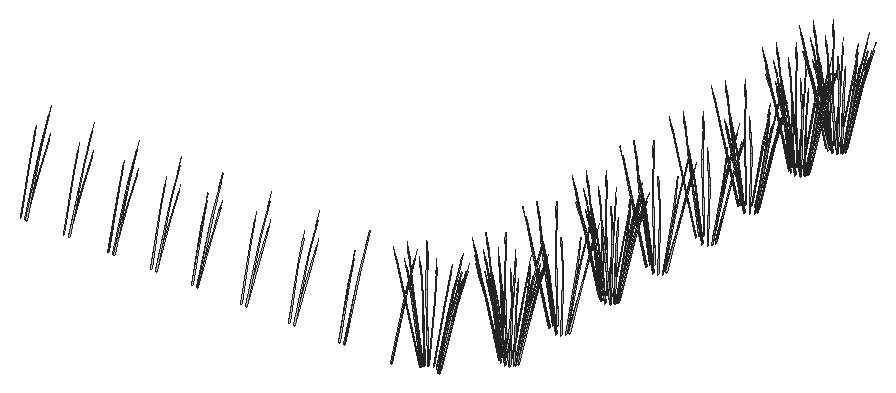
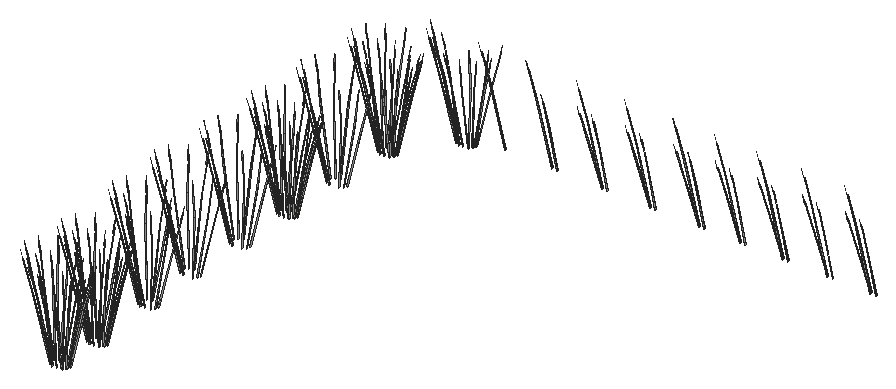
# SketchUp Ruby script. Lengths in inches.
U = 1.inch
M = Sketchup.active_model
def pt(a) = Geom::Point3d.new(a.map { |v| v * U })
def face(e, loops, mat)
  f = e.add_face(loops[0].map { |a| pt(a) })
  loops[1..].each { |l| e.add_face(l.map { |a| pt(a) }).erase! }
  f.material = f.back_material = mat if mat
  f
end
# faces: each face lists its corners as indices into pts; further lists are holes
def faces(e, pts, list, mat = nil) = list.each { |f| face(e, (f[0].is_a?(Array) ? f : [f]).map { |l| l.map { |i| pts[i] } }, mat) }
# xy, xz, yz: faces in a plane at the given z, y or x. An outline is a flat list of corners, or four numbers for a rectangle; further outlines are holes
def ring(l) = l.size == 4 ? [[l[0], l[1]], [l[2], l[1]], [l[2], l[3]], [l[0], l[3]]] : l.each_slice(2).to_a
def flat(e, list, mat, &to3) = list.each { |f| face(e, (f[0].is_a?(Array) ? f : [f]).map { |l| ring(l).map { |u, v| to3.(u, v) } }, mat) }
def xy(e, z, list, mat = nil) = flat(e, list, mat) { |x, y| [x, y, z] }
def xz(e, y, list, mat = nil) = flat(e, list, mat) { |x, z| [x, y, z] }
def yz(e, x, list, mat = nil) = flat(e, list, mat) { |y, z| [x, y, z] }
def lines(e, pts, list) = list.each { |a, b| e.add_line(pt(pts[a]), pt(pts[b])) }
# prism: a flat outline (further loops are holes) pulled along v
def prism(e, loops, v, mat = nil)
  f = face(e, loops, mat); d = Geom::Vector3d.new(v.map { |x| x * U })
  f.pushpull(f.normal.samedirection?(d) ? d.length : -d.length)
end
def box(e, o, s, mat = nil) = prism(e, [[o, [o[0] + s[0], o[1], o[2]], [o[0] + s[0], o[1] + s[1], o[2]], [o[0], o[1] + s[1], o[2]]]], [0, 0, s[2]], mat)
def at(x, y, z, deg = 0) = Geom::Transformation.translation(pt([x, y, z])) * Geom::Transformation.rotation(ORIGIN, Z_AXIS, deg.degrees)
def axes(o, x, y, z) = Geom::Transformation.new([*x, 0, *y, 0, *z, 0, *pt(o).to_a, 1])
def part(name) = M.definitions.add(name)
# library, detail: a bought-in or finely detailed component or shape, given as its bounding box
def library(name, o, s) = part(name).tap { |d| box(d.entities, o, s) }
def detail(e, o, s) = box(e.add_group.entities, o, s)
def put(e, d, t, mat = nil) = e.add_instance(d, t).tap { |i| i.material = mat if mat }
def group(e, t, mat = nil) = e.add_group.tap { |g| g.transformation = t; g.material = mat if mat }.entities
root = M.entities
M.materials.add("LightPink_Translucent").color = [144, 107, 117]
M.materials["LightPink_Translucent"].alpha = 0.75
c1 = part("blade")
p = [[2.15,0.21,22],[0,0.17,0],[0.09,0.45,0],[2.18,0.31,22],[2.29,0.31,22],[0.38,0.45,0],
  [2.48,0.24,33],[2.49,0.24,33],[2.48,0.22,33]]
faces(c1.entities,p,[[0,1,2,3],[4,5,2,3],[6,3,4,7],[8,0,3,6]])
c2 = part("seeds")
p = [[0.3,-0.1,1.38],[-0.01,-0.03,1.59],[-0.01,-0.03,0.03],[0.14,-0.07,-0.07],[0.29,-0.03,3],[0.15,0.01,3.11]]
faces(c2.entities,p,[[0,1,2,3],[1,0,4,5]],"LightPink_Translucent")
c3 = part("blade with seeds")
put(c3.entities,c1,at(0,0,0))
put(c3.entities,c2,axes([2.4,0.25,30.99],[1.5799,-0.05474,1.17369],[-0.12525,1.92788,0.29478],[-0.07173,-0.02425,1.56792]))
put(root,c3,axes([346.88,56.26,259.73],[-0.34533,0.38816,0.0643],[-0.49176,-0.22599,0.50621],[0.15898,0.12445,0.77189]))
put(root,c3,axes([328.97,56.26,259.73],[-0.34533,0.38816,0.0643],[-0.49176,-0.22599,0.50621],[0.15898,0.12445,0.77189]))
put(root,c3,axes([310.87,56.26,259.73],[-0.34533,0.38816,0.0643],[-0.49176,-0.22599,0.50621],[0.15898,0.12445,0.77189]))
put(root,c3,axes([295.42,56.26,259.73],[-0.34533,0.38816,0.0643],[-0.49176,-0.22599,0.50621],[0.15898,0.12445,0.77189]))
put(root,c3,axes([279.69,56.26,259.73],[-0.34533,0.38816,0.0643],[-0.49176,-0.22599,0.50621],[0.15898,0.12445,0.77189]))
put(root,c3,axes([262.96,56.26,259.73],[-0.34533,0.38816,0.0643],[-0.49176,-0.22599,0.50621],[0.15898,0.12445,0.77189]))
put(root,c3,axes([246.9,56.26,259.73],[-0.34533,0.38816,0.0643],[-0.49176,-0.22599,0.50621],[0.15898,0.12445,0.77189]))
put(root,c3,axes([397.37,60.31,260.05],[-0.63144,-0.17046,0.35414],[0.18417,-0.49731,-0.4572],[0.25423,-0.0456,0.87481]))
put(root,c3,axes([383.44,56.15,259.73],[-0.75571,0.14023,0.48003],[-0.13115,-0.55007,0.3958],[0.17773,0.16212,0.9933]))
put(root,c3,axes([365.81,56.15,259.73],[-0.75571,0.14023,0.48003],[-0.13115,-0.55007,0.3958],[0.17773,0.16212,0.9933]))
put(root,c3,axes([347.03,56.15,259.73],[-0.75571,0.14023,0.48003],[-0.13115,-0.55007,0.3958],[0.17773,0.16212,0.9933]))
put(root,c3,axes([329.12,56.15,259.73],[-0.75571,0.14023,0.48003],[-0.13115,-0.55007,0.3958],[0.17773,0.16212,0.9933]))
put(root,c3,axes([311.01,56.15,259.73],[-0.75571,0.14023,0.48003],[-0.13115,-0.55007,0.3958],[0.17773,0.16212,0.9933]))
put(root,c3,axes([295.5625,56.15,259.73],[-0.75571,0.14023,0.48003],[-0.13115,-0.55007,0.3958],[0.17773,0.16212,0.9933]))
put(root,c3,axes([279.84,56.15,259.73],[-0.75571,0.14023,0.48003],[-0.13115,-0.55007,0.3958],[0.17773,0.16212,0.9933]))
put(root,c3,axes([263.11,56.15,259.73],[-0.75571,0.14023,0.48003],[-0.13115,-0.55007,0.3958],[0.17773,0.16212,0.9933]))
put(root,c3,axes([247.04,56.15,259.73],[-0.75571,0.14023,0.48003],[-0.13115,-0.55007,0.3958],[0.17773,0.16212,0.9933]))
put(root,c3,axes([390.76,59.4,259.73],[0.21466,-0.55714,0.48003],[0.70573,0.19051,0.3958],[-0.27753,0.03348,0.9933]))
put(root,c3,axes([363.75,56.32,259.73],[-0.55987,0.20767,0.0643],[-0.27403,-0.37869,0.50621],[0.05407,0.16693,0.77189]))
put(root,c3,axes([344.96,56.32,259.73],[-0.55987,0.20767,0.0643],[-0.27403,-0.37869,0.50621],[0.05407,0.16693,0.77189]))
put(root,c3,axes([327.06,56.32,259.73],[-0.55987,0.20767,0.0643],[-0.27403,-0.37869,0.50621],[0.05407,0.16693,0.77189]))
put(root,c3,axes([308.95,56.32,259.73],[-0.55987,0.20767,0.0643],[-0.27403,-0.37869,0.50621],[0.05407,0.16693,0.77189]))
put(root,c3,axes([293.5,56.32,259.73],[-0.55987,0.20767,0.0643],[-0.27403,-0.37869,0.50621],[0.05407,0.16693,0.77189]))
put(root,c3,axes([277.77,56.32,259.73],[-0.55987,0.20767,0.0643],[-0.27403,-0.37869,0.50621],[0.05407,0.16693,0.77189]))
put(root,c3,axes([261.04,56.32,259.73],[-0.55987,0.20767,0.0643],[-0.27403,-0.37869,0.50621],[0.05407,0.16693,0.77189]))
put(root,c3,axes([244.98,56.32,259.73],[-0.55987,0.20767,0.0643],[-0.27403,-0.37869,0.50621],[0.05407,0.16693,0.77189]))
put(root,c3,axes([397.89,60.3125,259.73],[-0.21466,0.55714,0.48003],[-0.70573,-0.19051,0.3958],[0.27753,-0.03348,0.9933]))
put(root,c3,axes([391.28,59.4,260.05],[0.63144,0.17046,0.35414],[-0.18417,0.49731,-0.4572],[-0.25423,0.0456,0.87481]))
put(root,c3,axes([396.66,61.38,260.05],[-0.43232,-0.38257,0.35414],[0.49364,-0.36215,-0.4572],[0.25081,0.0551,0.87481]))
put(root,c3,axes([390.93,60.78,259.73],[-0.18844,-0.56237,0.48003],[0.73919,-0.0976,0.3958],[-0.21785,0.13226,0.9933]))
put(root,c3,axes([391.39,60.6,260.05],[0.66138,-0.08733,0.35414],[0.17464,0.49921,-0.4572],[-0.18953,0.13408,0.87481]))
put(root,c3,axes([397.11,61.58,259.73],[-0.56024,0.40262,0.48003],[-0.48318,-0.42758,0.3958],[0.26285,0.07427,0.9933]))
put(root,c3,axes([395.32,62.04,260.05],[-0.11735,-0.49217,0.35414],[0.67083,-0.12996,-0.4572],[0.18018,0.14104,0.87481]))
put(root,c3,axes([392.28,61.59,260.05],[0.5141,-0.32171,0.35414],[0.48666,0.36734,-0.4572],[-0.07405,0.18664,0.87481]))
put(root,c3,axes([392.01,61.92,259.73],[-0.54105,-0.41691,0.48003],[0.57458,-0.35956,0.3958],[-0.0998,0.1956,0.9933]))
put(root,c3,axes([393.72,62.12,260.05],[0.22906,-0.4699,0.35414],[0.66828,0.13705,-0.4572],[0.06128,0.18919,0.87481]))
put(root,c3,axes([395.58,62.38,259.73],[-0.75571,0.14023,0.48003],[-0.13115,-0.55007,0.3958],[0.17773,0.16212,0.9933]))
put(root,c3,axes([409.56,75.64,259.73],[0.74868,0.15974,0.48003],[-0.25601,0.52518,0.3958],[-0.04499,-0.20653,0.9933]))
put(root,c3,axes([409.55,76.02,260.05],[-0.22906,0.4699,0.35414],[-0.66828,-0.13705,-0.4572],[-0.06128,-0.18919,0.87481]))
put(root,c3,axes([411.26,76.22,259.73],[0.54105,0.41691,0.48003],[-0.57458,0.35956,0.3958],[0.0998,-0.1956,0.9933]))
put(root,c3,axes([410.99,76.55,260.05],[-0.5141,0.32171,0.35414],[-0.48666,-0.36734,-0.4572],[0.07405,-0.18664,0.87481]))
put(root,c3,axes([407.94,76.1,260.05],[0.11735,0.49217,0.35414],[-0.67083,0.12996,-0.4572],[-0.18018,-0.14104,0.87481]))
put(root,c3,axes([411.88,77.55,260.05],[-0.66138,0.08733,0.35414],[-0.17464,-0.49921,-0.4572],[0.18953,-0.13408,0.87481]))
put(root,c3,axes([412.34,77.36,259.73],[0.18844,0.56237,0.48003],[-0.73919,0.0976,0.3958],[0.21785,-0.13226,0.9933]))
put(root,c3,axes([406.61,76.77,260.05],[0.43232,0.38257,0.35414],[-0.49364,0.36215,-0.4572],[-0.25081,-0.0551,0.87481]))
put(root,c3,axes([411.99,78.74,260.05],[-0.63144,-0.17046,0.35414],[0.18417,-0.49731,-0.4572],[0.25423,-0.0456,0.87481]))
put(root,c3,axes([405.38,77.83,259.73],[0.21466,-0.55714,0.48003],[0.70573,0.19051,0.3958],[-0.27753,0.03348,0.9933]))
put(root,c3,axes([412.51,78.75,259.73],[-0.21466,0.55714,0.48003],[-0.70573,-0.19051,0.3958],[0.27753,-0.03348,0.9933]))
put(root,c3,axes([405.9,77.84,260.05],[0.63144,0.17046,0.35414],[-0.18417,0.49731,-0.4572],[-0.25423,0.0456,0.87481]))
put(root,c3,axes([411.28,79.8125,260.05],[-0.43232,-0.38257,0.35414],[0.49364,-0.36215,-0.4572],[0.25081,0.0551,0.87481]))
put(root,c3,axes([405.55,79.22,259.73],[-0.18844,-0.56237,0.48003],[0.73919,-0.0976,0.3958],[-0.21785,0.13226,0.9933]))
put(root,c3,axes([406,79.03,260.05],[0.66138,-0.08733,0.35414],[0.17464,0.49921,-0.4572],[-0.18953,0.13408,0.87481]))
put(root,c3,axes([411.72,80.01,259.73],[-0.56024,0.40262,0.48003],[-0.48318,-0.42758,0.3958],[0.26285,0.07427,0.9933]))
put(root,c3,axes([409.94,80.48,260.05],[-0.11735,-0.49217,0.35414],[0.67083,-0.12996,-0.4572],[0.18018,0.14104,0.87481]))
put(root,c3,axes([406.89,80.03,260.05],[0.5141,-0.32171,0.35414],[0.48666,0.36734,-0.4572],[-0.07405,0.18664,0.87481]))
put(root,c3,axes([406.63,80.36,259.73],[-0.54105,-0.41691,0.48003],[0.57458,-0.35956,0.3958],[-0.0998,0.1956,0.9933]))
put(root,c3,axes([408.34,80.56,260.05],[0.22906,-0.4699,0.35414],[0.66828,0.13705,-0.4572],[0.06128,0.18919,0.87481]))
put(root,c3,axes([410.19,80.81,259.73],[-0.75571,0.14023,0.48003],[-0.13115,-0.55007,0.3958],[0.17773,0.16212,0.9933]))
put(root,c3,axes([409.68,99.16,259.73],[0.74868,0.15974,0.48003],[-0.25601,0.52518,0.3958],[-0.04499,-0.20653,0.9933]))
put(root,c3,axes([411.38,99.75,259.73],[0.54105,0.41691,0.48003],[-0.57458,0.35956,0.3958],[0.0998,-0.1956,0.9933]))
put(root,c3,axes([412.46,100.89,259.73],[0.18844,0.56237,0.48003],[-0.73919,0.0976,0.3958],[0.21785,-0.13226,0.9933]))
put(root,c3,axes([405.5,101.36,259.73],[0.21466,-0.55714,0.48003],[0.70573,0.19051,0.3958],[-0.27753,0.03348,0.9933]))
put(root,c3,axes([412.63,102.27,259.73],[-0.21466,0.55714,0.48003],[-0.70573,-0.19051,0.3958],[0.27753,-0.03348,0.9933]))
put(root,c3,axes([405.67,102.74,259.73],[-0.18844,-0.56237,0.48003],[0.73919,-0.0976,0.3958],[-0.21785,0.13226,0.9933]))
put(root,c3,axes([411.85,103.54,259.73],[-0.56024,0.40262,0.48003],[-0.48318,-0.42758,0.3958],[0.26285,0.07427,0.9933]))
put(root,c3,axes([406.75,103.88,259.73],[-0.54105,-0.41691,0.48003],[0.57458,-0.35956,0.3958],[-0.0998,0.1956,0.9933]))
put(root,c3,axes([410.32,104.34,259.73],[-0.75571,0.14023,0.48003],[-0.13115,-0.55007,0.3958],[0.17773,0.16212,0.9933]))
put(root,c3,axes([409.46,122.55,259.73],[0.74868,0.15974,0.48003],[-0.25601,0.52518,0.3958],[-0.04499,-0.20653,0.9933]))
put(root,c3,axes([409.46,122.94,260.05],[-0.22906,0.4699,0.35414],[-0.66828,-0.13705,-0.4572],[-0.06128,-0.18919,0.87481]))
put(root,c3,axes([411.16,123.13,259.73],[0.54105,0.41691,0.48003],[-0.57458,0.35956,0.3958],[0.0998,-0.1956,0.9933]))
put(root,c3,axes([410.9,123.46,260.05],[-0.5141,0.32171,0.35414],[-0.48666,-0.36734,-0.4572],[0.07405,-0.18664,0.87481]))
put(root,c3,axes([407.85,123.01,260.05],[0.11735,0.49217,0.35414],[-0.67083,0.12996,-0.4572],[-0.18018,-0.14104,0.87481]))
put(root,c3,axes([411.79,124.46,260.05],[-0.66138,0.08733,0.35414],[-0.17464,-0.49921,-0.4572],[0.18953,-0.13408,0.87481]))
put(root,c3,axes([412.24,124.27,259.73],[0.18844,0.56237,0.48003],[-0.73919,0.0976,0.3958],[0.21785,-0.13226,0.9933]))
put(root,c3,axes([406.51,123.68,260.05],[0.43232,0.38257,0.35414],[-0.49364,0.36215,-0.4572],[-0.25081,-0.0551,0.87481]))
put(root,c3,axes([411.9,125.65,260.05],[-0.63144,-0.17046,0.35414],[0.18417,-0.49731,-0.4572],[0.25423,-0.0456,0.87481]))
put(root,c3,axes([405.28,124.74,259.73],[0.21466,-0.55714,0.48003],[0.70573,0.19051,0.3958],[-0.27753,0.03348,0.9933]))
put(root,c3,axes([412.41,125.66,259.73],[-0.21466,0.55714,0.48003],[-0.70573,-0.19051,0.3958],[0.27753,-0.03348,0.9933]))
put(root,c3,axes([405.8,124.75,260.05],[0.63144,0.17046,0.35414],[-0.18417,0.49731,-0.4572],[-0.25423,0.0456,0.87481]))
put(root,c3,axes([411.18,126.73,260.05],[-0.43232,-0.38257,0.35414],[0.49364,-0.36215,-0.4572],[0.25081,0.0551,0.87481]))
put(root,c3,axes([405.45,126.13,259.73],[-0.18844,-0.56237,0.48003],[0.73919,-0.0976,0.3958],[-0.21785,0.13226,0.9933]))
put(root,c3,axes([405.91,125.94,260.05],[0.66138,-0.08733,0.35414],[0.17464,0.49921,-0.4572],[-0.18953,0.13408,0.87481]))
put(root,c3,axes([411.63,126.92,259.73],[-0.56024,0.40262,0.48003],[-0.48318,-0.42758,0.3958],[0.26285,0.07427,0.9933]))
put(root,c3,axes([409.85,127.39,260.05],[-0.11735,-0.49217,0.35414],[0.67083,-0.12996,-0.4572],[0.18018,0.14104,0.87481]))
put(root,c3,axes([406.8,126.9375,260.05],[0.5141,-0.32171,0.35414],[0.48666,0.36734,-0.4572],[-0.07405,0.18664,0.87481]))
put(root,c3,axes([406.53,127.27,259.73],[-0.54105,-0.41691,0.48003],[0.57458,-0.35956,0.3958],[-0.0998,0.1956,0.9933]))
put(root,c3,axes([408.24,127.47,260.05],[0.22906,-0.4699,0.35414],[0.66828,0.13705,-0.4572],[0.06128,0.18919,0.87481]))
put(root,c3,axes([410.1,127.73,259.73],[-0.75571,0.14023,0.48003],[-0.13115,-0.55007,0.3958],[0.17773,0.16212,0.9933]))
put(root,c3,axes([409.1875,144.96,259.73],[0.74868,0.15974,0.48003],[-0.25601,0.52518,0.3958],[-0.04499,-0.20653,0.9933]))
put(root,c3,axes([410.89,145.54,259.73],[0.54105,0.41691,0.48003],[-0.57458,0.35956,0.3958],[0.0998,-0.1956,0.9933]))
put(root,c3,axes([411.97,146.68,259.73],[0.18844,0.56237,0.48003],[-0.73919,0.0976,0.3958],[0.21785,-0.13226,0.9933]))
put(root,c3,axes([405.01,147.15,259.73],[0.21466,-0.55714,0.48003],[0.70573,0.19051,0.3958],[-0.27753,0.03348,0.9933]))
put(root,c3,axes([412.14,148.07,259.73],[-0.21466,0.55714,0.48003],[-0.70573,-0.19051,0.3958],[0.27753,-0.03348,0.9933]))
put(root,c3,axes([405.18,148.54,259.73],[-0.18844,-0.56237,0.48003],[0.73919,-0.0976,0.3958],[-0.21785,0.13226,0.9933]))
put(root,c3,axes([411.35,149.33,259.73],[-0.56024,0.40262,0.48003],[-0.48318,-0.42758,0.3958],[0.26285,0.07427,0.9933]))
put(root,c3,axes([406.26,149.68,259.73],[-0.54105,-0.41691,0.48003],[0.57458,-0.35956,0.3958],[-0.0998,0.1956,0.9933]))
put(root,c3,axes([409.82,150.14,259.73],[-0.75571,0.14023,0.48003],[-0.13115,-0.55007,0.3958],[0.17773,0.16212,0.9933]))
put(root,c3,axes([409.55,167.55,259.73],[0.74868,0.15974,0.48003],[-0.25601,0.52518,0.3958],[-0.04499,-0.20653,0.9933]))
put(root,c3,axes([411.25,168.14,259.73],[0.54105,0.41691,0.48003],[-0.57458,0.35956,0.3958],[0.0998,-0.1956,0.9933]))
put(root,c3,axes([412.33,169.28,259.73],[0.18844,0.56237,0.48003],[-0.73919,0.0976,0.3958],[0.21785,-0.13226,0.9933]))
put(root,c3,axes([405.37,169.75,259.73],[0.21466,-0.55714,0.48003],[0.70573,0.19051,0.3958],[-0.27753,0.03348,0.9933]))
put(root,c3,axes([412.5,170.66,259.73],[-0.21466,0.55714,0.48003],[-0.70573,-0.19051,0.3958],[0.27753,-0.03348,0.9933]))
put(root,c3,axes([405.54,171.14,259.73],[-0.18844,-0.56237,0.48003],[0.73919,-0.0976,0.3958],[-0.21785,0.13226,0.9933]))
put(root,c3,axes([411.71,171.93,259.73],[-0.56024,0.40262,0.48003],[-0.48318,-0.42758,0.3958],[0.26285,0.07427,0.9933]))
put(root,c3,axes([406.62,172.27,259.73],[-0.54105,-0.41691,0.48003],[0.57458,-0.35956,0.3958],[-0.0998,0.1956,0.9933]))
put(root,c3,axes([410.18,172.73,259.73],[-0.75571,0.14023,0.48003],[-0.13115,-0.55007,0.3958],[0.17773,0.16212,0.9933]))
put(root,c3,axes([407.53,189.68,259.73],[0.74868,0.15974,0.48003],[-0.25601,0.52518,0.3958],[-0.04499,-0.20653,0.9933]))
put(root,c3,axes([407.52,190.07,260.05],[-0.22906,0.4699,0.35414],[-0.66828,-0.13705,-0.4572],[-0.06128,-0.18919,0.87481]))
put(root,c3,axes([409.23,190.27,259.73],[0.54105,0.41691,0.48003],[-0.57458,0.35956,0.3958],[0.0998,-0.1956,0.9933]))
put(root,c3,axes([410.31,191.41,259.73],[0.18844,0.56237,0.48003],[-0.73919,0.0976,0.3958],[0.21785,-0.13226,0.9933]))
put(root,c3,axes([409.96,192.79,260.05],[-0.63144,-0.17046,0.35414],[0.18417,-0.49731,-0.4572],[0.25423,-0.0456,0.87481]))
put(root,c3,axes([403.35,191.88,259.73],[0.21466,-0.55714,0.48003],[0.70573,0.19051,0.3958],[-0.27753,0.03348,0.9933]))
put(root,c3,axes([410.48,192.79,259.73],[-0.21466,0.55714,0.48003],[-0.70573,-0.19051,0.3958],[0.27753,-0.03348,0.9933]))
put(root,c3,axes([409.25,193.86,260.05],[-0.43232,-0.38257,0.35414],[0.49364,-0.36215,-0.4572],[0.25081,0.0551,0.87481]))
put(root,c3,axes([403.52,193.27,259.73],[-0.18844,-0.56237,0.48003],[0.73919,-0.0976,0.3958],[-0.21785,0.13226,0.9933]))
put(root,c3,axes([409.69,194.06,259.73],[-0.56024,0.40262,0.48003],[-0.48318,-0.42758,0.3958],[0.26285,0.07427,0.9933]))
put(root,c3,axes([404.6,194.4,259.73],[-0.54105,-0.41691,0.48003],[0.57458,-0.35956,0.3958],[-0.0998,0.1956,0.9933]))
put(root,c3,axes([406.31,194.6,260.05],[0.22906,-0.4699,0.35414],[0.66828,0.13705,-0.4572],[0.06128,0.18919,0.87481]))
put(root,c3,axes([408.16,194.86,259.73],[-0.75571,0.14023,0.48003],[-0.13115,-0.55007,0.3958],[0.17773,0.16212,0.9933]))
put(root,c3,axes([405.125,216.4375,259.73],[0.74868,0.15974,0.48003],[-0.25601,0.52518,0.3958],[-0.04499,-0.20653,0.9933]))
put(root,c3,axes([405.12,216.82,260.05],[-0.22906,0.4699,0.35414],[-0.66828,-0.13705,-0.4572],[-0.06128,-0.18919,0.87481]))
put(root,c3,axes([406.83,217.02,259.73],[0.54105,0.41691,0.48003],[-0.57458,0.35956,0.3958],[0.0998,-0.1956,0.9933]))
put(root,c3,axes([406.56,217.35,260.05],[-0.5141,0.32171,0.35414],[-0.48666,-0.36734,-0.4572],[0.07405,-0.18664,0.87481]))
put(root,c3,axes([403.51,216.9,260.05],[0.11735,0.49217,0.35414],[-0.67083,0.12996,-0.4572],[-0.18018,-0.14104,0.87481]))
put(root,c3,axes([407.45,218.35,260.05],[-0.66138,0.08733,0.35414],[-0.17464,-0.49921,-0.4572],[0.18953,-0.13408,0.87481]))
put(root,c3,axes([407.91,218.16,259.73],[0.18844,0.56237,0.48003],[-0.73919,0.0976,0.3958],[0.21785,-0.13226,0.9933]))
put(root,c3,axes([402.18,217.57,260.05],[0.43232,0.38257,0.35414],[-0.49364,0.36215,-0.4572],[-0.25081,-0.0551,0.87481]))
put(root,c3,axes([407.56,219.54,260.05],[-0.63144,-0.17046,0.35414],[0.18417,-0.49731,-0.4572],[0.25423,-0.0456,0.87481]))
put(root,c3,axes([400.95,218.63,259.73],[0.21466,-0.55714,0.48003],[0.70573,0.19051,0.3958],[-0.27753,0.03348,0.9933]))
put(root,c3,axes([408.08,219.55,259.73],[-0.21466,0.55714,0.48003],[-0.70573,-0.19051,0.3958],[0.27753,-0.03348,0.9933]))
put(root,c3,axes([401.46,218.64,260.05],[0.63144,0.17046,0.35414],[-0.18417,0.49731,-0.4572],[-0.25423,0.0456,0.87481]))
put(root,c3,axes([406.85,220.61,260.05],[-0.43232,-0.38257,0.35414],[0.49364,-0.36215,-0.4572],[0.25081,0.0551,0.87481]))
put(root,c3,axes([401.12,220.02,259.73],[-0.18844,-0.56237,0.48003],[0.73919,-0.0976,0.3958],[-0.21785,0.13226,0.9933]))
put(root,c3,axes([401.57,219.83,260.05],[0.66138,-0.08733,0.35414],[0.17464,0.49921,-0.4572],[-0.18953,0.13408,0.87481]))
put(root,c3,axes([407.29,220.8125,259.73],[-0.56024,0.40262,0.48003],[-0.48318,-0.42758,0.3958],[0.26285,0.07427,0.9933]))
put(root,c3,axes([405.51,221.28,260.05],[-0.11735,-0.49217,0.35414],[0.67083,-0.12996,-0.4572],[0.18018,0.14104,0.87481]))
put(root,c3,axes([402.46,220.83,260.05],[0.5141,-0.32171,0.35414],[0.48666,0.36734,-0.4572],[-0.07405,0.18664,0.87481]))
put(root,c3,axes([402.2,221.16,259.73],[-0.54105,-0.41691,0.48003],[0.57458,-0.35956,0.3958],[-0.0998,0.1956,0.9933]))
put(root,c3,axes([403.9,221.36,260.05],[0.22906,-0.4699,0.35414],[0.66828,0.13705,-0.4572],[0.06128,0.18919,0.87481]))
put(root,c3,axes([405.76,221.62,259.73],[-0.75571,0.14023,0.48003],[-0.13115,-0.55007,0.3958],[0.17773,0.16212,0.9933]))
put(root,c3,axes([405.28,233.51,259.73],[0.74868,0.15974,0.48003],[-0.25601,0.52518,0.3958],[-0.04499,-0.20653,0.9933]))
put(root,c3,axes([405.28,233.89,260.05],[-0.22906,0.4699,0.35414],[-0.66828,-0.13705,-0.4572],[-0.06128,-0.18919,0.87481]))
put(root,c3,axes([406.98,234.09,259.73],[0.54105,0.41691,0.48003],[-0.57458,0.35956,0.3958],[0.0998,-0.1956,0.9933]))
put(root,c3,axes([406.72,234.42,260.05],[-0.5141,0.32171,0.35414],[-0.48666,-0.36734,-0.4572],[0.07405,-0.18664,0.87481]))
put(root,c3,axes([403.67,233.97,260.05],[0.11735,0.49217,0.35414],[-0.67083,0.12996,-0.4572],[-0.18018,-0.14104,0.87481]))
put(root,c3,axes([407.61,235.42,260.05],[-0.66138,0.08733,0.35414],[-0.17464,-0.49921,-0.4572],[0.18953,-0.13408,0.87481]))
put(root,c3,axes([408.0625,235.23,259.73],[0.18844,0.56237,0.48003],[-0.73919,0.0976,0.3958],[0.21785,-0.13226,0.9933]))
put(root,c3,axes([402.33,234.64,260.05],[0.43232,0.38257,0.35414],[-0.49364,0.36215,-0.4572],[-0.25081,-0.0551,0.87481]))
put(root,c3,axes([407.72,236.61,260.05],[-0.63144,-0.17046,0.35414],[0.18417,-0.49731,-0.4572],[0.25423,-0.0456,0.87481]))
put(root,c3,axes([401.1,235.7,259.73],[0.21466,-0.55714,0.48003],[0.70573,0.19051,0.3958],[-0.27753,0.03348,0.9933]))
put(root,c3,axes([408.23,236.62,259.73],[-0.21466,0.55714,0.48003],[-0.70573,-0.19051,0.3958],[0.27753,-0.03348,0.9933]))
put(root,c3,axes([401.625,235.71,260.05],[0.63144,0.17046,0.35414],[-0.18417,0.49731,-0.4572],[-0.25423,0.0456,0.87481]))
put(root,c3,axes([407,237.68,260.05],[-0.43232,-0.38257,0.35414],[0.49364,-0.36215,-0.4572],[0.25081,0.0551,0.87481]))
put(root,c3,axes([401.27,237.09,259.73],[-0.18844,-0.56237,0.48003],[0.73919,-0.0976,0.3958],[-0.21785,0.13226,0.9933]))
put(root,c3,axes([401.73,236.9,260.05],[0.66138,-0.08733,0.35414],[0.17464,0.49921,-0.4572],[-0.18953,0.13408,0.87481]))
put(root,c3,axes([407.45,237.88,259.73],[-0.56024,0.40262,0.48003],[-0.48318,-0.42758,0.3958],[0.26285,0.07427,0.9933]))
put(root,c3,axes([405.67,238.35,260.05],[-0.11735,-0.49217,0.35414],[0.67083,-0.12996,-0.4572],[0.18018,0.14104,0.87481]))
put(root,c3,axes([402.62,237.9,260.05],[0.5141,-0.32171,0.35414],[0.48666,0.36734,-0.4572],[-0.07405,0.18664,0.87481]))
put(root,c3,axes([402.35,238.23,259.73],[-0.54105,-0.41691,0.48003],[0.57458,-0.35956,0.3958],[-0.0998,0.1956,0.9933]))
put(root,c3,axes([404.0625,238.43,260.05],[0.22906,-0.4699,0.35414],[0.66828,0.13705,-0.4572],[0.06128,0.18919,0.87481]))
put(root,c3,axes([405.92,238.6875,259.73],[-0.75571,0.14023,0.48003],[-0.13115,-0.55007,0.3958],[0.17773,0.16212,0.9933]))
